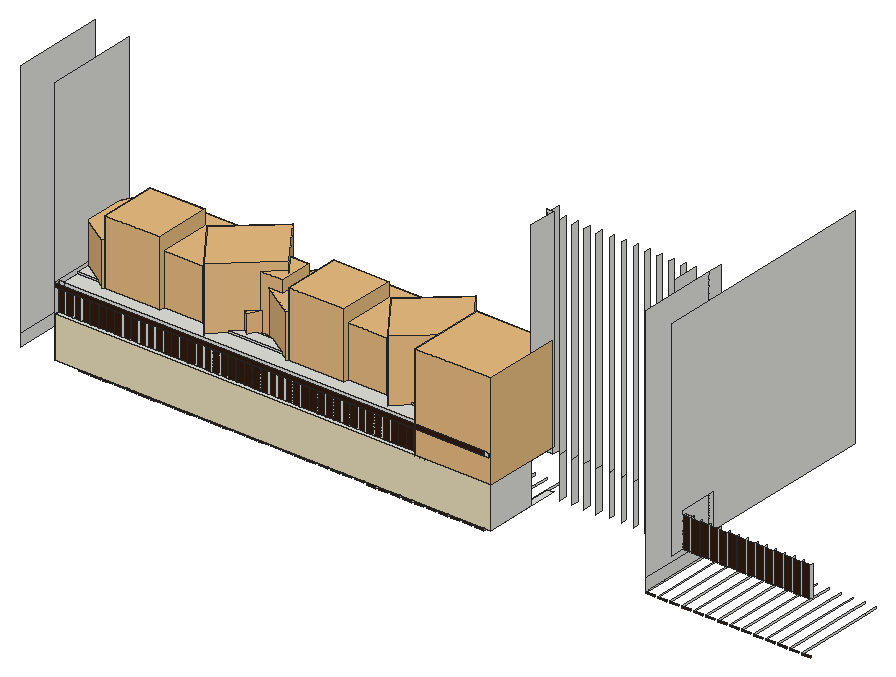
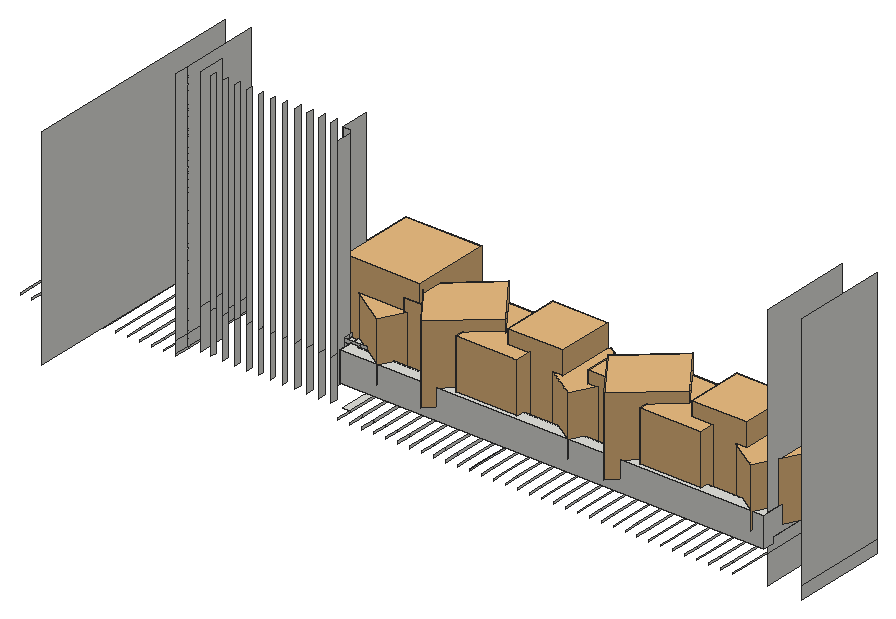
# SketchUp Ruby script. Lengths in inches.
U = 1.inch
M = Sketchup.active_model
def pt(a) = Geom::Point3d.new(a.map { |v| v * U })
def face(e, loops, mat)
  f = e.add_face(loops[0].map { |a| pt(a) })
  loops[1..].each { |l| e.add_face(l.map { |a| pt(a) }).erase! }
  f.material = f.back_material = mat if mat
  f
end
# faces: each face lists its corners as indices into pts; further lists are holes
def faces(e, pts, list, mat = nil) = list.each { |f| face(e, (f[0].is_a?(Array) ? f : [f]).map { |l| l.map { |i| pts[i] } }, mat) }
# xy, xz, yz: faces in a plane at the given z, y or x. An outline is a flat list of corners, or four numbers for a rectangle; further outlines are holes
def ring(l) = l.size == 4 ? [[l[0], l[1]], [l[2], l[1]], [l[2], l[3]], [l[0], l[3]]] : l.each_slice(2).to_a
def flat(e, list, mat, &to3) = list.each { |f| face(e, (f[0].is_a?(Array) ? f : [f]).map { |l| ring(l).map { |u, v| to3.(u, v) } }, mat) }
def xy(e, z, list, mat = nil) = flat(e, list, mat) { |x, y| [x, y, z] }
def xz(e, y, list, mat = nil) = flat(e, list, mat) { |x, z| [x, y, z] }
def yz(e, x, list, mat = nil) = flat(e, list, mat) { |y, z| [x, y, z] }
def lines(e, pts, list) = list.each { |a, b| e.add_line(pt(pts[a]), pt(pts[b])) }
# prism: a flat outline (further loops are holes) pulled along v
def prism(e, loops, v, mat = nil)
  f = face(e, loops, mat); d = Geom::Vector3d.new(v.map { |x| x * U })
  f.pushpull(f.normal.samedirection?(d) ? d.length : -d.length)
end
def box(e, o, s, mat = nil) = prism(e, [[o, [o[0] + s[0], o[1], o[2]], [o[0] + s[0], o[1] + s[1], o[2]], [o[0], o[1] + s[1], o[2]]]], [0, 0, s[2]], mat)
def at(x, y, z, deg = 0) = Geom::Transformation.translation(pt([x, y, z])) * Geom::Transformation.rotation(ORIGIN, Z_AXIS, deg.degrees)
def axes(o, x, y, z) = Geom::Transformation.new([*x, 0, *y, 0, *z, 0, *pt(o).to_a, 1])
def part(name) = M.definitions.add(name)
# library, detail: a bought-in or finely detailed component or shape, given as its bounding box
def library(name, o, s) = part(name).tap { |d| box(d.entities, o, s) }
def detail(e, o, s) = box(e.add_group.entities, o, s)
def put(e, d, t, mat = nil) = e.add_instance(d, t).tap { |i| i.material = mat if mat }
def group(e, t, mat = nil) = e.add_group.tap { |g| g.transformation = t; g.material = mat if mat }.entities
root = M.entities
M.materials.add("Material__1").color = [95, 70, 46]
M.materials.add("[Color D01]").color = [237, 225, 189]
M.materials.add("[Wood Veneer 01]").color = [51, 28, 15]
c1 = library("Areca palm plant",[0,0,0],[49.1,36.6,54.46])
c2 = library("Group\#74",[-84.69,-90.07,-0.36],[176.51,175.13,171.4])
c3 = library("Group20\#1",[-20.81,-17.08,3.79],[39.86,39.43,37.51])
c4 = library("Group\#130",[-7.34,-1.2,0],[38.67,35.81,49.04])
c5 = library("Group38\#2",[14.01,28.44,-23.43],[18.58,18.32,38.89])
c6 = part("Group\#16")
put(c6.entities,c1,axes([-6.2,158.41,6.08],[0.45017,-0.56191,0],[0.66137,0.52986,0],[0,0,0.72]))
put(c6.entities,c1,axes([-6.2,56.6,6.08],[0.45017,-0.56191,0],[0.66137,0.52986,0],[0,0,0.72]))
put(c6.entities,c2,axes([14.93,145.87,6.05],[-0.04961,-0.08593,0],[0.08593,-0.04961,0],[0,0,0.10522]))
put(c6.entities,c3,axes([18.97,79.98,4.77],[0,0.85,0],[-0.85,0,0],[0,0,0.85]))
put(c6.entities,c2,axes([14.93,173.12,6.05],[-0.04961,-0.08593,0],[0.08593,-0.04961,0],[0,0,0.10522]))
put(c6.entities,c2,axes([14.93,193.18,6.05],[-0.04961,-0.08593,0],[0.08593,-0.04961,0],[0,0,0.10522]))
put(c6.entities,c4,axes([24.9375,89.91,8],[0,0.79,0],[-0.79,0,0],[0,0,0.79]))
put(c6.entities,c5,axes([-4.1,-1.15,28.17],[0.8848,0,0],[0,0.94674,0],[0,0,0.85826]))
g1 = group(c6.entities,at(0,0,0))
xy(g1,0,[[0,0,6,234.8],[30,0,36,234.8]])
xy(g1,3,[[6,0,30,234.8]])
xy(g1,7,[[6,5,30,229.8]],"Material__1")
xy(g1,15,[[[0,0,36,234.8],[6,5,30,229.8]]])
xz(g1,0,[[0,0,6,0,6,3,30,3,30,0,36,0,36,15,0,15]])
xz(g1,5,[[6,7,30,15]])
xz(g1,229.8,[[6,7,30,15]])
xz(g1,234.8,[[0,0,0,15,36,15,36,0,30,0,30,3,6,3,6,0]])
yz(g1,0,[[0,0,234.8,15]])
yz(g1,6,[[0,0,234.8,3],[5,7,229.8,15]])
yz(g1,30,[[0,0,234.8,3],[5,7,229.8,15]])
yz(g1,36,[[0,0,234.8,15]])
put(c6.entities,c2,axes([14.93,91.37,6.05],[-0.04961,-0.08593,0],[0.08593,-0.04961,0],[0,0,0.10522]))
put(c6.entities,c2,axes([14.93,44.05,6.05],[-0.04961,-0.08593,0],[0.08593,-0.04961,0],[0,0,0.10522]))
put(c6.entities,c4,axes([24.9375,191.72,8],[0,0.79,0],[-0.79,0,0],[0,0,0.79]))
put(c6.entities,c5,axes([-4.1,100.66,28.17],[0.8848,0,0],[0,0.94674,0],[0,0,0.85826]))
put(c6.entities,c2,axes([17.19,15.79,6.07],[-0.08133,-0.14087,0],[0.14087,-0.08133,0],[0,0,0.1725]))
put(c6.entities,c2,axes([14.93,71.3,6.05],[-0.04961,-0.08593,0],[0.08593,-0.04961,0],[0,0,0.10522]))
put(c6.entities,c2,axes([17.19,121.23,6.07],[-0.08133,-0.14087,0],[0.14087,-0.08133,0],[0,0,0.1725]))
put(c6.entities,c2,axes([17.19,223.04,6.07],[-0.08133,-0.14087,0],[0.14087,-0.08133,0],[0,0,0.1725]))
put(c6.entities,c3,axes([18.97,181.79,4.77],[0,0.85,0],[-0.85,0,0],[0,0,0.85]))
c7 = library("plant (1)",[-35.72,-28.42,0],[66.31,67.39,84.38])
xy(root,254.6875,[[315.43,246.64,318.81,286.21]])
xy(root,269.0625,[[100.18,253.58,100.18,271.8,301.9,271.8,301.9,290.02,308.99,290.02,308.99,253.58]])
xy(root,275.125,[[100.18,246.64,318.81,249.27],[100.18,249.27,315.43,253.58],[315.43,249.27,318.81,253.58],[308.99,253.58,315.43,290.02],[315.43,253.58,318.81,286.21],
  [409.32,253.84,413.01,255.47]])
xy(root,287.25,[[100.18,246.64,315.43,249.27],[315.43,246.64,318.0625,249.27],[100.18,249.27,100.18,271.8,301.9,271.8,301.9,290.02,315.43,290.02,315.43,249.27],[315.43,249.27,318.0625,286.21]])
xz(root,246.64,[[244.68,254.625,249.43,254.6875],[315.43,287.25,318.0625,289.1875]])
xz(root,246.64,[[100.18,254.6875,318.81,275.125]],"[Color D01]")
xz(root,246.64,[[256.68,253.5625,261.43,254.6875],[262.68,253.5625,267.43,254.6875],[268.68,253.5625,273.43,254.6875],[274.68,253.5625,279.43,254.6875],[280.68,253.5625,285.43,254.6875],
  [286.68,253.5625,291.43,254.6875],[292.68,253.5625,297.43,254.6875],[298.68,253.5625,303.43,254.6875],[304.68,253.5625,309.43,254.6875],[310.68,253.5625,315.43,254.6875],
  [244.68,253.875,249.43,254.625],[250.68,253.875,255.43,254.6875],[112.68,253.9375,117.43,254.6875],[118.68,253.9375,123.43,254.6875],[124.68,253.9375,129.43,254.6875],
  [130.68,253.9375,135.43,254.6875],[136.68,253.9375,141.43,254.6875],[142.68,253.9375,147.43,254.6875],[148.68,253.9375,153.43,254.6875],[154.68,253.9375,159.43,254.6875],
  [160.68,253.9375,165.43,254.6875],[166.68,253.9375,171.43,254.6875],[172.68,253.9375,177.43,254.6875],[178.68,253.9375,183.43,254.6875],[184.68,253.9375,189.43,254.6875],
  [190.68,253.9375,195.43,254.6875],[196.68,253.9375,201.43,254.6875],[202.68,253.9375,207.43,254.6875],[208.68,253.9375,213.43,254.6875],[214.68,253.9375,219.43,254.6875],
  [220.68,253.9375,225.43,254.6875],[226.68,253.9375,231.43,254.6875],[232.68,253.9375,237.43,254.6875],[238.68,253.9375,243.43,254.6875],[396.57,253.9375,400.96,254.6875],
  [402.57,253.9375,406.96,254.6875],[408.57,253.9375,412.96,254.6875],[414.57,253.9375,418.96,254.6875],[420.57,253.9375,424.96,254.6875],[426.57,253.9375,430.96,254.6875],
  [432.57,253.9375,436.96,254.6875],[438.57,253.9375,442.96,254.6875],[444.57,253.9375,448.96,254.6875],[450.57,253.9375,454.96,254.6875],[456.57,253.9375,460.96,254.6875],
  [462.57,253.9375,466.96,254.6875],[468.57,253.9375,472.96,254.6875],[474.57,253.9375,478.96,254.6875],[100.18,287.25,315.43,289.1875]],"[Wood Veneer 01]")
xz(root,249.27,[[103.45,275.125,104.24,287.25],[107.52,275.125,108.3,287.25],[111.58,275.125,112.36,287.25],[115.64,275.125,116.43,287.25],[119.7,275.125,120.49,287.25],
  [123.77,275.125,124.55,287.25],[127.83,275.125,128.61,287.25],[131.89,275.125,132.68,287.25],[135.95,275.125,136.74,287.25],[140.02,275.125,140.8,287.25],
  [144.08,275.125,144.86,287.25],[148.14,275.125,148.93,287.25],[152.2,275.125,152.99,287.25],[156.27,275.125,157.05,287.25],[160.33,275.125,161.11,287.25],
  [164.39,275.125,165.18,287.25],[168.45,275.125,169.24,287.25],[172.52,275.125,173.3,287.25],[176.58,275.125,177.36,287.25],[180.64,275.125,181.43,287.25],
  [184.7,275.125,185.49,287.25],[188.77,275.125,189.55,287.25],[192.83,275.125,193.61,287.25],[196.89,275.125,197.68,287.25],[200.95,275.125,201.74,287.25],
  [205.02,275.125,205.8,287.25],[209.08,275.125,209.86,287.25],[213.14,275.125,213.93,287.25],[217.2,275.125,217.99,287.25],[221.27,275.125,222.05,287.25],
  [225.33,275.125,226.11,287.25],[229.39,275.125,230.18,287.25],[233.45,275.125,234.24,287.25],[237.52,275.125,238.3,287.25],[241.58,275.125,242.36,287.25],
  [245.64,275.125,246.43,287.25],[249.7,275.125,250.49,287.25],[253.77,275.125,254.55,287.25],[257.83,275.125,258.61,287.25],[261.89,275.125,262.68,287.25],
  [265.95,275.125,266.74,287.25],[270.02,275.125,270.8,287.25],[274.08,275.125,274.86,287.25],[278.14,275.125,278.93,287.25],[282.2,275.125,282.99,287.25],
  [286.27,275.125,287.05,287.25],[290.33,275.125,291.11,287.25],[294.39,275.125,295.18,287.25],[298.45,275.125,299.24,287.25],[302.52,275.125,303.3,287.25],
  [306.58,275.125,307.36,287.25],[310.64,275.125,311.43,287.25],[314.7,275.125,315.43,287.25],[100.18,287.25,103.45,289.1875],[103.45,287.25,315.43,289.1875],
  [315.43,287.25,318.0625,289.1875]])
xz(root,249.27,[[100.18,275.125,103.45,287.25],[104.24,275.125,107.52,287.25],[108.3,275.125,111.58,287.25],[112.36,275.125,115.64,287.25],[116.43,275.125,119.7,287.25],
  [120.49,275.125,123.77,287.25],[124.55,275.125,127.83,287.25],[128.61,275.125,131.89,287.25],[132.68,275.125,135.95,287.25],[136.74,275.125,140.02,287.25],
  [140.8,275.125,144.08,287.25],[144.86,275.125,148.14,287.25],[148.93,275.125,152.2,287.25],[152.99,275.125,156.27,287.25],[157.05,275.125,160.33,287.25],
  [161.11,275.125,164.39,287.25],[165.18,275.125,168.45,287.25],[169.24,275.125,172.52,287.25],[173.3,275.125,176.58,287.25],[177.36,275.125,180.64,287.25],
  [181.43,275.125,184.7,287.25],[185.49,275.125,188.77,287.25],[189.55,275.125,192.83,287.25],[193.61,275.125,196.89,287.25],[197.68,275.125,200.95,287.25],
  [201.74,275.125,205.02,287.25],[205.8,275.125,209.08,287.25],[209.86,275.125,213.14,287.25],[213.93,275.125,217.2,287.25],[217.99,275.125,221.27,287.25],
  [222.05,275.125,225.33,287.25],[226.11,275.125,229.39,287.25],[230.18,275.125,233.45,287.25],[234.24,275.125,237.52,287.25],[238.3,275.125,241.58,287.25],
  [242.36,275.125,245.64,287.25],[246.43,275.125,249.7,287.25],[250.49,275.125,253.77,287.25],[254.55,275.125,257.83,287.25],[258.61,275.125,261.89,287.25],
  [262.68,275.125,265.95,287.25],[266.74,275.125,270.02,287.25],[270.8,275.125,274.08,287.25],[274.86,275.125,278.14,287.25],[278.93,275.125,282.2,287.25],
  [282.99,275.125,286.27,287.25],[287.05,275.125,290.33,287.25],[291.11,275.125,294.39,287.25],[295.18,275.125,298.45,287.25],[299.24,275.125,302.52,287.25],
  [303.3,275.125,306.58,287.25],[307.36,275.125,310.64,287.25],[311.43,275.125,314.7,287.25]],"[Wood Veneer 01]")
xz(root,253.58,[[100.18,269.0625,308.99,275.125]])
xz(root,253.84,[[409.32,275.125,413.01,290.375],[413.95,275.125,417.64,290.375],[418.57,275.125,422.26,290.375],[423.2,275.125,426.89,290.375],[427.82,275.125,431.51,290.375],
  [432.45,275.125,436.14,290.375],[437.07,275.125,440.76,290.375],[441.7,275.125,445.39,290.375],[446.32,275.125,450.01,290.375],[450.95,275.125,454.64,290.375],
  [455.57,275.125,459.26,290.375],[460.2,275.125,463.89,290.375],[464.82,275.125,468.51,290.375],[469.45,275.125,473.14,290.375]],"[Wood Veneer 01]")
xz(root,255.47,[[409.32,275.125,413.01,290.375]])
xz(root,271.8,[[100.18,269.0625,301.9,287.25],[100.18,287.25,301.9,289.1875]])
xz(root,286.21,[[315.43,275.125,318.81,275.125,318.81,380.6875,315.43,380.6875,315.43,289.1875,318.0625,289.1875,318.0625,287.25,315.43,287.25],[315.43,287.25,318.0625,289.1875]])
xz(root,290.02,[[301.9,269.0625,301.9,287.25,315.43,287.25,315.43,275.125,308.99,275.125,308.99,269.0625],[308.99,269.0625,315.43,275.125],[301.9,287.25,315.43,289.1875]])
yz(root,83.125,[[246.64,254.6875,293.46,260.6875],[246.64,260.6875,293.46,380.6875]])
yz(root,100.18,[[246.64,254.6875,293.46,254.6875,293.46,269.0625,253.58,269.0625,253.58,275.125,246.64,275.125],[253.58,269.0625,271.8,275.125],[271.8,269.0625,293.46,275.125],[246.64,275.125,249.27,287.25],[271.8,275.125,293.46,275.125,293.46,378.875,246.64,378.875,246.64,289.1875,271.8,289.1875],
  [249.27,275.125,271.8,287.25],[246.64,287.25,249.27,289.1875],[249.27,287.25,271.8,289.1875]])
yz(root,117.43,[[246.64,253.9375,286.21,254.6875],[286.21,253.9375,293.45,254.6875]])
yz(root,123.43,[[246.64,253.9375,286.21,254.6875],[286.21,253.9375,293.45,254.6875]])
yz(root,129.43,[[246.64,253.9375,286.21,254.6875],[286.21,253.9375,293.45,254.6875]])
yz(root,135.43,[[246.64,253.9375,286.21,254.6875],[286.21,253.9375,293.45,254.6875]])
yz(root,141.43,[[246.64,253.9375,286.21,254.6875],[286.21,253.9375,293.45,254.6875]])
yz(root,147.43,[[246.64,253.9375,286.21,254.6875],[286.21,253.9375,293.45,254.6875]])
yz(root,153.43,[[246.64,253.9375,286.21,254.6875],[286.21,253.9375,293.45,254.6875]])
yz(root,159.43,[[246.64,253.9375,286.21,254.6875],[286.21,253.9375,293.45,254.6875]])
yz(root,165.43,[[246.64,253.9375,286.21,254.6875],[286.21,253.9375,293.45,254.6875]])
yz(root,171.43,[[246.64,253.9375,286.21,254.6875],[286.21,253.9375,293.45,254.6875]])
yz(root,177.43,[[246.64,253.9375,286.21,254.6875],[286.21,253.9375,293.45,254.6875]])
yz(root,183.43,[[246.64,253.9375,286.21,254.6875],[286.21,253.9375,293.45,254.6875]])
yz(root,189.43,[[246.64,253.9375,286.21,254.6875],[286.21,253.9375,293.45,254.6875]])
yz(root,195.43,[[246.64,253.9375,286.21,254.6875],[286.21,253.9375,293.45,254.6875]])
yz(root,201.43,[[246.64,253.9375,286.21,254.6875],[286.21,253.9375,293.45,254.6875]])
yz(root,207.43,[[246.64,253.9375,286.21,254.6875],[286.21,253.9375,293.45,254.6875]])
yz(root,213.43,[[246.64,253.9375,286.21,254.6875],[286.21,253.9375,293.45,254.6875]])
yz(root,219.43,[[246.64,253.9375,286.21,254.6875],[286.21,253.9375,293.45,254.6875]])
yz(root,225.43,[[246.64,253.9375,286.21,254.6875],[286.21,253.9375,293.45,254.6875]])
yz(root,231.43,[[246.64,253.9375,286.21,254.6875],[286.21,253.9375,293.45,254.6875]])
yz(root,237.43,[[246.64,253.9375,286.21,254.6875],[286.21,253.9375,293.45,254.6875]])
yz(root,243.43,[[246.64,253.9375,286.21,254.6875],[286.21,253.9375,293.45,254.6875]])
yz(root,249.43,[[246.64,253.875,286.21,254.625],[286.21,253.875,293.45,254.625],[246.64,254.625,286.21,254.6875],[286.21,254.625,293.45,254.6875]])
yz(root,255.43,[[246.64,253.875,286.21,254.6875],[286.21,253.875,293.45,254.6875]])
yz(root,261.43,[[246.64,253.5625,286.21,254.6875],[286.21,253.5625,293.45,254.6875]])
yz(root,267.43,[[246.64,253.5625,286.21,254.6875],[286.21,253.5625,293.45,254.6875]])
yz(root,273.43,[[246.64,253.5625,286.21,254.6875],[286.21,253.5625,293.45,254.6875]])
yz(root,279.43,[[246.64,253.5625,286.21,254.6875],[286.21,253.5625,293.45,254.6875]])
yz(root,285.43,[[246.64,253.5625,286.21,254.6875],[286.21,253.5625,293.45,254.6875]])
yz(root,291.43,[[246.64,253.5625,286.21,254.6875],[286.21,253.5625,293.45,254.6875]])
yz(root,297.43,[[246.64,253.5625,286.21,254.6875],[286.21,253.5625,293.45,254.6875]])
yz(root,301.9,[[271.8,269.0625,290.02,287.25],[271.8,287.25,290.02,289.1875]])
yz(root,303.43,[[246.64,253.5625,286.21,254.6875],[286.21,253.5625,293.45,254.6875]])
yz(root,308.99,[[253.58,269.0625,290.02,275.125]])
yz(root,309.43,[[246.64,253.5625,286.21,254.6875],[286.21,253.5625,293.45,254.6875]])
yz(root,315.43,[[246.64,253.5625,286.21,254.6875],[286.21,253.5625,293.45,254.6875],[290.02,269.0625,290.02,289.1875,286.21,289.1875,286.21,378.875,293.45,378.875,293.45,269.0625],[249.27,275.125,286.21,287.25],[286.21,275.125,290.02,287.25],
  [246.64,287.25,249.27,289.1875],[249.27,287.25,286.21,289.1875],[286.21,287.25,290.02,289.1875]])
yz(root,318.0625,[[246.64,287.25,249.27,289.1875],[249.27,287.25,286.21,289.1875]])
yz(root,318.81,[[246.64,254.6875,271.96,275.125],[271.96,275.125,286.21,380.6875]])
yz(root,324.81,[[282.52,254.6875,286.21,275.125],[282.52,275.125,286.21,380.6875]])
yz(root,330.81,[[282.52,254.6875,286.21,275.125],[282.52,275.125,286.21,380.6875]])
yz(root,336.81,[[282.52,254.6875,286.21,275.125],[282.52,275.125,286.21,380.6875]])
yz(root,342.81,[[282.52,254.6875,286.21,275.125],[282.52,275.125,286.21,380.6875]])
yz(root,348.81,[[283.46,254.6875,286.21,275.125],[283.46,275.125,286.21,380.6875]])
yz(root,354.81,[[283.46,254.6875,286.21,275.125],[283.46,275.125,286.21,380.6875]])
yz(root,360.81,[[283.46,254.6875,286.21,275.125],[283.46,275.125,286.21,380.6875]])
yz(root,366.81,[[283.46,254.6875,286.21,275.125],[283.46,275.125,286.21,380.6875]])
yz(root,372.81,[[283.46,254.6875,286.21,275.125],[283.46,275.125,286.21,380.6875]])
yz(root,378.81,[[283.46,254.6875,286.21,275.125],[283.46,275.125,286.21,380.6875]])
yz(root,384.81,[[283.46,254.6875,286.21,275.125],[283.46,275.125,286.21,380.6875]])
yz(root,390.12,[[272.89,254.6875,286.21,275.125],[272.89,275.125,286.21,380.6875]])
yz(root,396.57,[[246.64,253.9375,286.21,254.6875],[286.21,253.9375,293.45,254.6875],[246.64,254.6875,286.21,260.6875],[286.21,254.6875,293.45,260.6875],[246.64,260.6875,286.21,380.6875],
  [286.21,260.6875,293.45,380.6875]])
yz(root,402.57,[[246.64,253.9375,286.21,254.6875],[286.21,253.9375,293.45,254.6875]])
yz(root,408.57,[[246.64,253.9375,286.21,254.6875],[286.21,253.9375,293.45,254.6875]])
yz(root,409.32,[[246.64,275.125,253.84,275.125,253.84,290.375,253.22,290.375,253.22,292.5625,273.33,292.5625,273.33,275.125,361.27,275.125,361.27,379.5625,246.64,379.5625],[253.84,275.125,255.47,290.375]])
yz(root,413.01,[[253.84,275.125,255.47,290.375],[255.47,275.125,255.84,290.375]])
yz(root,414.57,[[246.64,253.9375,286.21,254.6875],[286.21,253.9375,293.45,254.6875]])
yz(root,417.64,[[253.84,275.125,255.47,290.375]])
yz(root,420.57,[[246.64,253.9375,286.21,254.6875],[286.21,253.9375,293.45,254.6875]])
yz(root,422.26,[[253.84,275.125,255.47,290.375]])
yz(root,426.57,[[246.64,253.9375,286.21,254.6875],[286.21,253.9375,293.45,254.6875]])
yz(root,426.89,[[253.84,275.125,255.47,290.375]])
yz(root,431.51,[[253.84,275.125,255.47,290.375]])
yz(root,432.57,[[246.64,253.9375,286.21,254.6875],[286.21,253.9375,293.45,254.6875]])
yz(root,436.14,[[253.84,275.125,255.47,290.375]])
yz(root,438.57,[[246.64,253.9375,286.21,254.6875],[286.21,253.9375,293.45,254.6875]])
yz(root,440.76,[[253.84,275.125,255.47,290.375]])
yz(root,444.57,[[246.64,253.9375,286.21,254.6875],[286.21,253.9375,293.45,254.6875]])
yz(root,445.39,[[253.84,275.125,255.47,290.375]])
yz(root,450.01,[[253.84,275.125,255.47,290.375]])
yz(root,450.57,[[246.64,253.9375,286.21,254.6875],[286.21,253.9375,293.45,254.6875]])
yz(root,454.64,[[253.84,275.125,255.47,290.375]])
yz(root,456.57,[[246.64,253.9375,286.21,254.6875],[286.21,253.9375,293.45,254.6875]])
yz(root,459.26,[[253.84,275.125,255.47,290.375]])
yz(root,462.57,[[246.64,253.9375,286.21,254.6875],[286.21,253.9375,293.45,254.6875]])
yz(root,463.89,[[253.84,275.125,255.47,290.375]])
yz(root,468.51,[[253.84,275.125,255.47,290.375]])
yz(root,468.57,[[246.64,253.9375,286.21,254.6875],[286.21,253.9375,293.45,254.6875]])
yz(root,473.14,[[253.84,275.125,255.47,290.375]])
yz(root,474.57,[[246.64,253.9375,286.21,254.6875],[286.21,253.9375,293.45,254.6875]])
put(root,c6,axes([311.76,260.97,273.05],[0,1,0],[-0.9045,0,0],[0,0,1]))
put(root,c7,axes([301.375,262.85,275.125],[0.57,0,0],[0,0.57,0],[0,0,0.57]))
